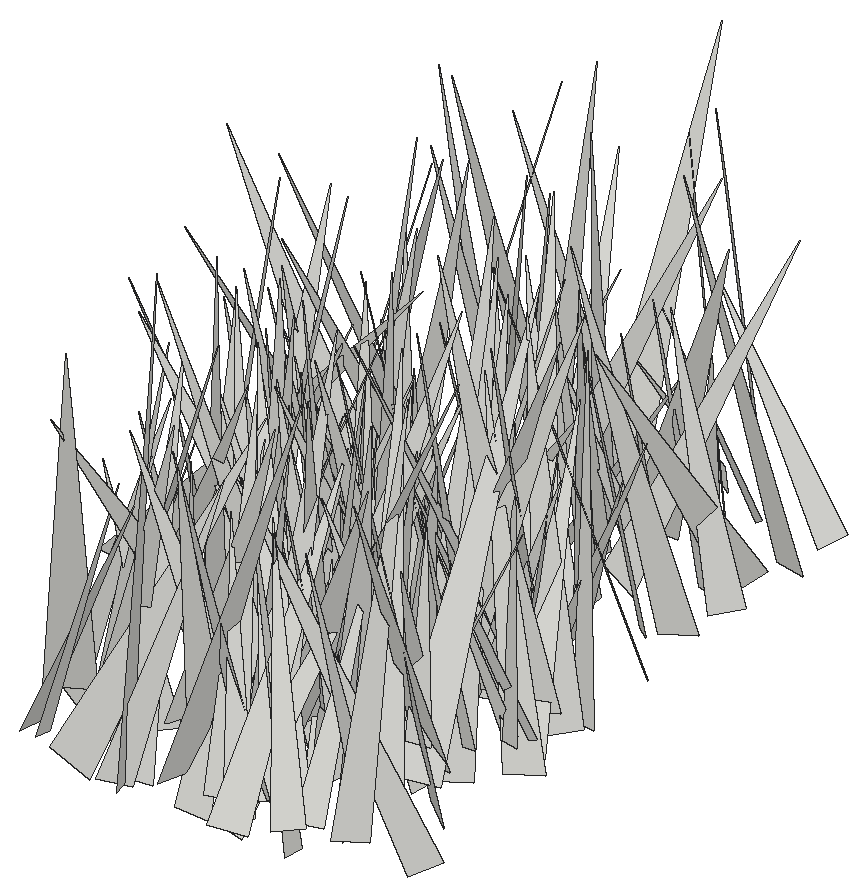
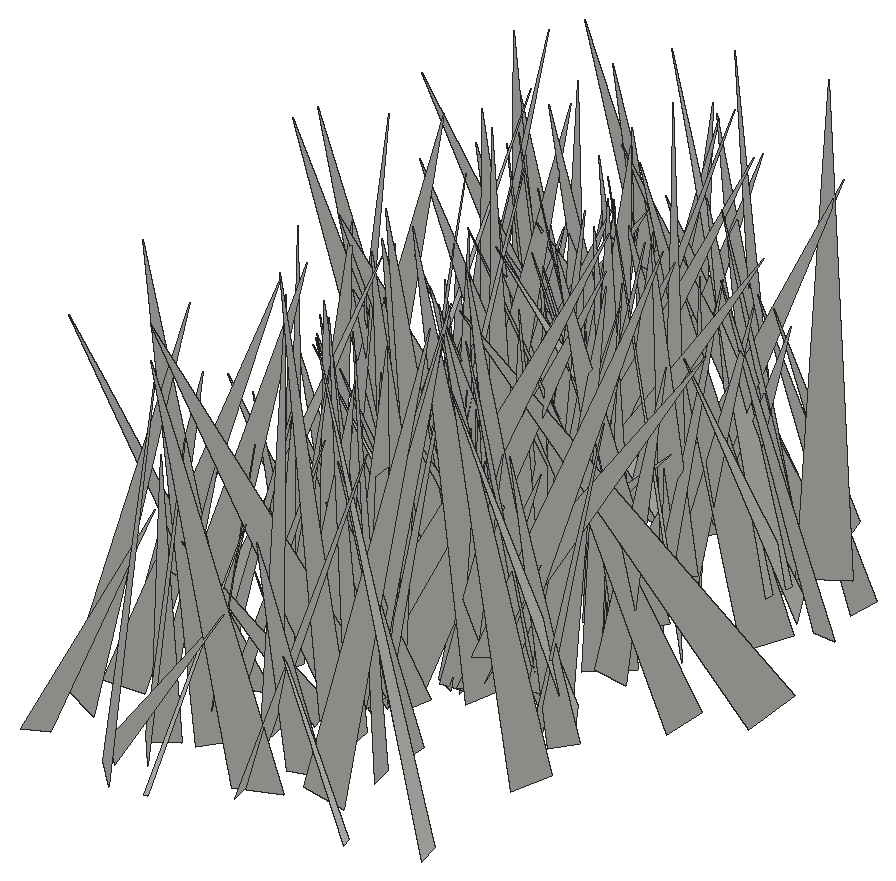
# SketchUp Ruby script. Lengths in inches.
U = 1.inch
M = Sketchup.active_model
def pt(a) = Geom::Point3d.new(a.map { |v| v * U })
def face(e, loops, mat)
  f = e.add_face(loops[0].map { |a| pt(a) })
  loops[1..].each { |l| e.add_face(l.map { |a| pt(a) }).erase! }
  f.material = f.back_material = mat if mat
  f
end
# faces: each face lists its corners as indices into pts; further lists are holes
def faces(e, pts, list, mat = nil) = list.each { |f| face(e, (f[0].is_a?(Array) ? f : [f]).map { |l| l.map { |i| pts[i] } }, mat) }
# xy, xz, yz: faces in a plane at the given z, y or x. An outline is a flat list of corners, or four numbers for a rectangle; further outlines are holes
def ring(l) = l.size == 4 ? [[l[0], l[1]], [l[2], l[1]], [l[2], l[3]], [l[0], l[3]]] : l.each_slice(2).to_a
def flat(e, list, mat, &to3) = list.each { |f| face(e, (f[0].is_a?(Array) ? f : [f]).map { |l| ring(l).map { |u, v| to3.(u, v) } }, mat) }
def xy(e, z, list, mat = nil) = flat(e, list, mat) { |x, y| [x, y, z] }
def xz(e, y, list, mat = nil) = flat(e, list, mat) { |x, z| [x, y, z] }
def yz(e, x, list, mat = nil) = flat(e, list, mat) { |y, z| [x, y, z] }
def lines(e, pts, list) = list.each { |a, b| e.add_line(pt(pts[a]), pt(pts[b])) }
# prism: a flat outline (further loops are holes) pulled along v
def prism(e, loops, v, mat = nil)
  f = face(e, loops, mat); d = Geom::Vector3d.new(v.map { |x| x * U })
  f.pushpull(f.normal.samedirection?(d) ? d.length : -d.length)
end
def box(e, o, s, mat = nil) = prism(e, [[o, [o[0] + s[0], o[1], o[2]], [o[0] + s[0], o[1] + s[1], o[2]], [o[0], o[1] + s[1], o[2]]]], [0, 0, s[2]], mat)
def at(x, y, z, deg = 0) = Geom::Transformation.translation(pt([x, y, z])) * Geom::Transformation.rotation(ORIGIN, Z_AXIS, deg.degrees)
def axes(o, x, y, z) = Geom::Transformation.new([*x, 0, *y, 0, *z, 0, *pt(o).to_a, 1])
def part(name) = M.definitions.add(name)
# library, detail: a bought-in or finely detailed component or shape, given as its bounding box
def library(name, o, s) = part(name).tap { |d| box(d.entities, o, s) }
def detail(e, o, s) = box(e.add_group.entities, o, s)
def put(e, d, t, mat = nil) = e.add_instance(d, t).tap { |i| i.material = mat if mat }
def group(e, t, mat = nil) = e.add_group.tap { |g| g.transformation = t; g.material = mat if mat }.entities
root = M.entities
c1 = part("fur_instance\#9")
p = [[0.8125,0,1.79],[0.67,-0.02,1.48],[0,-0.11,0],[0,0.11,0]]
faces(c1.entities,p,[[0,1,2,3]])
put(root,c1,axes([88.67,204.02,-27.1],[-0.10037,-5.00985,1.67679],[-5.24561,-0.10471,-0.62683],[-0.62754,1.67652,4.9715]))
put(root,c1,axes([86.56,196.72,-28.22],[2.54446,5.11145,1.43196],[5.2695,-2.24073,-1.36501],[0.64019,-1.87187,5.54418]))
put(root,c1,axes([88,208.36,-27.1],[-4.12038,-2.11418,1.50488],[-1.47976,4.23386,1.89649],[2.13184,-1.14743,4.225]))
put(root,c1,axes([83.72,202.71,-27.1],[6.0984,-4.54505,0.22334],[-3.82324,-4.91501,4.37303],[2.46783,3.61705,6.22291]))
put(root,c1,axes([87.83,206.67,-27.1],[5.27233,3.79468,0.9806],[3.62511,-5.34626,1.19781],[-1.48988,0.42019,6.38454]))
put(root,c1,axes([86.71,194.7,-28.22],[4.99939,-0.31235,0.02616],[-0.31267,-4.999,0.06629],[-0.02197,0.06779,5.0087]))
put(root,c1,axes([88.11,195.89,-28.22],[4.4489,2.71988,0.66857],[2.4928,-4.41728,1.38241],[-1.27698,0.85286,5.02786]))
put(root,c1,axes([91.18,206.82,-27.1],[-7.69272,2.37823,1.5322],[2.71051,7.46743,2.01798],[0.8104,-2.40066,7.79498]))
put(root,c1,axes([86.53,203.27,-28.22],[5.89255,-1.31891,0.46121],[-1.38894,-5.74659,1.31223],[-0.15186,1.38261,5.89404]))
put(root,c1,axes([87.44,195.62,-27.1],[4.02071,-6.30995,0.86141],[-6.36147,-4.02715,0.19326],[-0.29869,0.83076,7.47959]))
put(root,c1,axes([87.19,208.02,-27.1],[2.31724,-3.70248,0.25487],[-3.62607,-2.19471,1.08527],[0.79054,0.78602,4.23086]))
put(root,c1,axes([86.52,210.37,-27.1],[7.28234,-1.08518,0.65082],[-1.04869,-7.30325,-0.44316],[-0.70811,-0.34428,7.3494]))
put(root,c1,axes([92.48,206.29,-27.1],[-2.35699,-6.63901,0.53799],[-6.01099,1.87426,-3.2057],[-2.86948,1.52709,6.27339]))
put(root,c1,axes([86.24,215.52,-27.1],[7.20484,3.15988,1.15153],[3.35999,-6.88107,-2.14053],[-0.14588,-2.42624,7.57051]))
put(root,c1,axes([88.13,201.4,-27.1],[5.88152,4.86813,2.28116],[5.13014,-6.09312,-0.22398],[-1.60749,-1.63397,7.63157]))
put(root,c1,axes([88.56,192.9,-27.1],[4.03699,1.00135,1.00845],[0.75439,-4.0837,1.03503],[-1.2044,0.79854,4.02849]))
put(root,c1,axes([89.36,205.97,-27.1],[1.80262,-6.00522,1.15434],[-6.08405,-1.88243,-0.2921],[-0.61598,1.01901,6.26312]))
put(root,c1,axes([90.63,198.56,-28.22],[-1.01611,-5.1437,1.43202],[-5.3112,0.8243,-0.80778],[-0.54728,1.55038,5.1805]))
put(root,c1,axes([89.47,194.375,-27.1],[3.26782,5.25044,1.3347],[5.28581,-3.43164,0.55786],[-1.18691,-0.82697,6.1591]))
put(root,c1,axes([90.27,200.12,-28.22],[-3.05463,-4.97038,1.37571],[-5.09206,3.16016,0.11108],[0.81742,1.11209,5.83293]))
put(root,c1,axes([89.72,201.24,-27.1],[-4.86903,5.31705,1.90275],[5.12727,5.21523,-1.45307],[2.36698,-0.35954,7.06166]))
put(root,c1,axes([91.3,195.46,-27.1],[-1.35537,3.98703,1.26023],[4.07237,0.95801,1.34893],[-0.94888,-1.58348,3.98921]))
put(root,c1,axes([91.07,206.75,-27.1],[-3.67924,-0.76157,0.35539],[-0.68587,3.64327,0.70657],[0.48566,-0.62424,3.6902]))
put(root,c1,axes([90.7,214.8,-27.1],[-1.04582,-7.4675,1.55674],[-7.62212,0.96116,-0.50998],[-0.30029,1.61039,7.52311]))
put(root,c1,axes([90.63,204.97,-28.22],[4.06044,6.49572,1.60929],[6.19974,-4.35997,1.95581],[-2.5194,-0.26008,7.4065]))
put(root,c1,axes([90.6875,198.125,-28.22],[-0.28002,6.79198,1.74012],[7.00527,0.19856,0.35229],[-0.29175,-1.75129,6.78861]))
put(root,c1,axes([91.42,199.84,-28.22],[4.2838,-6.03866,0.74714],[-5.20831,-4.11147,-3.36808],[-3.14598,-1.41597,6.59337]))
put(root,c1,axes([89.03,202.06,-27.1],[-4.56158,-4.36485,4.54967],[-5.17144,5.80258,0.38189],[3.60662,2.79958,6.30192]))
put(root,c1,axes([88.56,216.4375,-27.1],[3.77978,1.93812,0.15141],[1.88384,-3.56988,-1.33157],[0.48001,-1.25124,4.0336]))
put(root,c1,axes([87.59,198.0625,-28.22],[6.5822,-3.48627,0.04021],[-3.46978,-6.5418,0.80411],[0.34104,0.72931,7.40492]))
put(root,c1,axes([90.8,201.92,-27.1],[-3.25997,-4.21096,1.97124],[-4.4396,3.53441,0.20814],[1.38129,1.42168,5.3213]))
put(root,c1,axes([91.86,202.38,-27.1],[-6.39617,-0.72322,1.67284],[-0.5993,6.59982,0.56183],[1.72113,-0.38959,6.41236]))
put(root,c1,axes([90.17,202.17,-28.22],[5.05478,-5.09898,2.04992],[-5.28407,-5.27475,-0.09077],[-1.51011,1.38923,7.17929]))
put(root,c1,axes([91.77,207.32,-27.1],[1.42744,-3.53628,2.17287],[-3.81125,-2.02664,-0.79456],[-1.64348,1.62839,3.72982]))
put(root,c1,axes([91.72,203.55,-28.22],[-4.92159,1.07561,1.43405],[1.22896,5.07505,0.41117],[1.30503,-0.72281,5.02095]))
put(root,c1,axes([91.13,193.9375,-28.22],[-0.62472,6.74476,1.37593],[6.88336,0.62526,0.06028],[0.06565,-1.37569,6.77336]))
put(root,c1,axes([92.85,215.76,-27.1],[-6.22564,-1.43503,0.72375],[-1.44178,6.26598,0.02194],[0.71021,0.14105,6.38885]))
put(root,c1,axes([90.58,198.62,-27.1],[7.19679,1.10507,2.93039],[1.40985,-7.70082,-0.55845],[-2.79655,-1.03845,7.25969]))
put(root,c1,axes([90.63,203.49,-27.1],[4.23333,1.58778,2.03705],[2.11026,-4.38143,-0.97034],[-1.48911,-1.69519,4.41595]))
put(root,c1,axes([92.93,204.93,-28.22],[-6.67208,0.88571,0.68005],[0.61302,6.34873,-2.25421],[0.93335,2.16166,6.3419]))
put(root,c1,axes([87.98,197.04,-27.1],[8.03575,1.73258,0.69022],[1.85682,-7.7181,-2.24381],[-0.17451,-2.34107,7.90825]))
put(root,c1,axes([93.67,209.41,-27.1],[1.68916,7.29229,2.94864],[7.0223,-2.75681,2.79508],[-3.5439,-1.98689,6.94394]))
put(root,c1,axes([90.39,201.42,-27.1],[5.9168,-1.45412,1.7202],[-1.44139,-6.15974,-0.24915],[-1.73089,0.15879,6.08776]))
put(root,c1,axes([89.06,195.42,-28.22],[2.07111,-6.85146,1.31632],[-6.80663,-1.68294,1.94991],[1.53132,1.78604,6.88693]))
put(root,c1,axes([90.87,201.98,-27.1],[-1.22041,-5.00142,1.71972],[-5.19067,1.47111,0.5948],[1.01418,1.51086,5.11369]))
put(root,c1,axes([91.99,214.01,-27.1],[-1.75814,5.2069,0.13379],[5.20853,1.75836,0.01288],[0.0306,-0.13088,5.4957]))
put(root,c1,axes([95.95,198.13,-28.22],[-5.6206,-6.05261,0.8091],[-5.56666,4.62654,-4.06048],[-2.5102,3.29256,7.1929]))
put(root,c1,axes([93.41,207.71,-27.1],[0.03934,-7.1777,0.79174],[-6.87762,-0.27857,-2.18369],[-2.20103,0.74216,6.83757]))
put(root,c1,axes([90.37,205.62,-27.1],[0.14436,6.2225,2.72909],[6.68972,0.34776,-1.14678],[1.18962,-2.71069,6.11762]))
put(root,c1,axes([91.48,196.51,-27.1],[-1.7362,-3.80786,1.79903],[-4.13168,1.91701,0.07019],[0.81577,1.60498,4.18441]))
put(root,c1,axes([91.21,201,-28.22],[2.09335,-3.21544,0.11512],[-3.16402,-2.08217,-0.6229],[-0.58423,-0.24481,3.78592]))
put(root,c1,axes([90.17,212.79,-27.1],[6.17791,2.14602,1.95241],[2.61385,-6.11017,-1.55482],[-1.25898,-2.15507,6.35252]))
put(root,c1,axes([93.86,201.84,-28.22],[-6.45817,-1.9042,0.82118],[-2.02073,6.38203,-1.093],[0.4658,1.28531,6.64374]))
put(root,c1,axes([94.68,200.33,-27.1],[-3.03964,-3.22245,0.08473],[-2.53096,2.3136,-2.80576],[-1.9964,1.97328,3.42802]))
put(root,c1,axes([92.28,203.53,-27.1],[-1.52023,5.3398,1.43684],[5.52962,1.4775,0.35965],[0.03531,-1.48075,5.54032]))
put(root,c1,axes([90.29,211.18,-27.1],[4.64255,0.07182,0.51653],[0.0806,-4.67045,-0.07504],[-0.51523,-0.08349,4.6425]))
put(root,c1,axes([95,206.625,-27.1],[-3.02685,-7.70536,1.30124],[-7.48247,2.45538,-2.86554],[-2.25353,2.19686,7.76679]))
put(root,c1,axes([92.36,192.05,-27.1],[-7.10447,-2.39928,3.44832],[-3.25719,7.42464,-1.54476],[2.65295,2.69055,7.33783]))
put(root,c1,axes([92.16,207.35,-27.1],[-1.43466,-3.23484,0.82707],[-3.31328,1.49057,0.08262],[0.41278,0.72144,3.53774]))
put(root,c1,axes([90.76,207.02,-27.1],[7.15421,-1.9799,2.12173],[-2.22149,-7.36827,0.61487],[-1.86728,1.18029,7.39761]))
put(root,c1,axes([89.07,193.55,-28.22],[0.42432,7.03314,2.02201],[6.63788,0.48281,-3.07232],[3.08094,-2.00885,6.34082]))
put(root,c1,axes([93.4,210.47,-27.1],[-1.73003,-6.76572,2.01517],[-7.01807,1.42401,-1.24409],[-0.76325,2.2419,6.8717]))
put(root,c1,axes([94.2,195.89,-27.1],[-0.66678,7.09806,0.59701],[6.83624,0.46921,2.05647],[-2.00116,-0.76214,6.82627]))
put(root,c1,axes([94.1,203.72,-28.22],[-3.14834,2.92622,0.07201],[2.87738,3.07451,0.86494],[-0.53726,-0.68166,4.21031]))
put(root,c1,axes([95.25,199.83,-28.22],[-7.87957,1.88276,1.17896],[2.17634,7.41366,2.70618],[0.44527,-2.91806,7.63603]))
put(root,c1,axes([94.67,198.18,-27.1],[-7.8071,-1.03462,1.04066],[-0.93299,7.84786,0.80297],[1.13267,-0.66693,7.83431]))
put(root,c1,axes([92.92,209.3,-27.1],[-2.78076,-3.999,1.01738],[-3.97731,2.92434,0.62365],[1.09912,0.46468,4.83071]))
put(root,c1,axes([91.3125,198.9,-28.22],[5.1332,2.66859,0.80867],[2.72409,-5.16107,-0.26035],[-0.59552,-0.60587,5.77956]))
put(root,c1,axes([91.71,195.98,-28.22],[6.02604,4.35688,0.13616],[4.14402,-5.7981,2.12678],[-1.35204,1.64734,7.12547]))
put(root,c1,axes([92.08,211.55,-27.1],[6.17707,1.48648,1.9777],[1.80034,-6.34915,-0.85095],[-1.69697,-1.32504,6.29616]))
put(root,c1,axes([92.28,205.46,-27.1],[3.64013,-0.49009,0.65042],[-0.33955,-3.62113,-0.82821],[-0.74023,-0.74902,3.57838]))
put(root,c1,axes([92.1,191.9,-27.1],[4.14579,-2.60609,2.17076],[-3.31381,-3.84297,1.71517],[-0.72292,2.67047,4.58667]))
put(root,c1,axes([92.86,211.54,-27.1],[2.51079,7.35519,2.45383],[7.71335,-2.63218,-0.00261],[-0.79014,-2.32314,7.77193]))
put(root,c1,axes([92.45,215.7,-27.1],[-1.03239,7.59334,1.92082],[7.72051,1.31303,-1.04105],[1.31985,-1.74108,7.59215]))
put(root,c1,axes([94.75,195.29,-27.1],[-5.48359,2.23586,1.70204],[2.68404,5.27249,1.72124],[0.83185,-2.27324,5.66623]))
put(root,c1,axes([93.9,199.51,-27.1],[3.52477,-3.78027,2.43443],[-3.94318,-4.08529,-0.63451],[-2.1606,1.28874,5.1295]))
put(root,c1,axes([96.17,197.18,-27.1],[-1.67581,5.69721,1.32161],[5.39716,0.9769,2.63242],[-2.25291,-1.89755,5.32325]))
put(root,c1,axes([94.71,199.63,-27.1],[-3.5063,-5.04513,2.56803],[-5.65565,3.25438,-1.32851],[0.24851,2.88062,5.99854]))
put(root,c1,axes([92.49,209.21,-27.1],[3.64505,-0.39812,0.27738],[-0.20845,-3.18305,-1.82936],[-0.43816,-1.79764,3.17779]))
put(root,c1,axes([93.27,201.86,-28.22],[4.67368,1.9817,0.84614],[1.46066,-4.3994,2.23565],[-1.58416,1.79011,4.55767]))
put(root,c1,axes([95.12,198.55,-27.1],[-3.33504,1.53851,0.16438],[1.54705,3.32218,0.29368],[0.02564,-0.33558,3.66104]))
put(root,c1,axes([95.26,201.24,-28.22],[0.65103,4.23875,0.31259],[3.78552,-0.72206,1.9071],[-1.9325,0.01355,3.84107]))
put(root,c1,axes([93.59,205.57,-27.1],[-2.68709,-2.60275,1.28992],[-2.48203,2.97011,0.82256],[1.50922,0.25052,3.6494]))
put(root,c1,axes([93.89,193.41,-28.22],[0.04484,6.03011,0.93276],[6.10111,-0.02998,-0.09948],[0.09373,-0.93336,6.02946]))
put(root,c1,axes([93.67,194.61,-27.1],[3.36896,-5.0045,1.18358],[-5.04079,-3.49374,-0.42432],[-1.01802,0.73793,6.01788]))
put(root,c1,axes([94.76,199.71,-28.22],[-5.05417,-1.27819,2.14403],[-1.86511,5.15169,-1.32541],[1.65892,1.89778,5.04199]))
put(root,c1,axes([94.18,212.875,-27.1],[-6.46976,-1.55499,2.98827],[-1.52534,7.12153,0.40334],[3.00351,0.26714,6.64177]))
put(root,c1,axes([92.61,198.42,-27.1],[3.5807,5.01538,0.32607],[5.01642,-3.54168,-0.61141],[0.30977,-0.61982,6.13202]))
put(root,c1,axes([91.86,195.84,-27.1],[3.71453,-6.09838,0.78607],[-6.05056,-3.46164,1.73599],[1.09493,1.55972,6.92635]))
put(root,c1,axes([93.44,201.57,-27.1],[4.01305,-1.4697,0.35123],[-1.33059,-3.90931,-1.15533],[-0.71618,-0.97223,4.11458]))
put(root,c1,axes([93.33,208.65,-27.1],[3.21105,-3.45107,0.18225],[-3.45172,-3.21492,-0.06213],[-0.16965,0.09106,4.71348]))
put(root,c1,axes([92.04,208.89,-27.1],[2.63596,-3.80697,0.02165],[-3.40971,-2.34911,2.07299],[1.69332,1.196,4.14053]))
put(root,c1,axes([93.87,196.59,-28.22],[3.27247,4.57721,0.86039],[4.6176,-3.3258,0.13012],[-0.60735,-0.62316,5.62521]))
put(root,c1,axes([94.32,201.8,-28.22],[7.55648,0.00384,2.83421],[0.13477,-8.06186,-0.34839],[-2.831,-0.37353,7.54844]))
put(root,c1,axes([96.33,208.05,-27.1],[-2.8304,4.89567,0.80261],[4.94903,2.72215,0.8485],[-0.34477,-1.11592,5.59096]))
put(root,c1,axes([95.92,194.07,-27.1],[-2.42816,-5.42807,1.43938],[-5.61543,2.33238,-0.67728],[-0.05217,1.5899,5.90772]))
put(root,c1,axes([95.34,193.2,-27.1],[-1.64071,6.20292,1.41522],[6.35653,1.66047,0.09149],[0.27128,-1.39198,6.41559]))
put(root,c1,axes([97.22,216.5,-27.1],[-2.6027,-3.00196,0.39616],[-2.70686,2.07255,-2.07851],[-1.35707,1.62343,3.38609]))
put(root,c1,axes([94.85,217.9,-27.1],[-2.93741,-3.09466,0.01129],[-2.71699,2.58635,2.03327],[1.48156,-1.39259,3.75115]))
put(root,c1,axes([96.63,201.31,-27.1],[1.14957,-5.99203,1.40359],[-5.68779,-1.57972,-2.08556],[-2.35023,0.89221,5.73379]))
put(root,c1,axes([96.74,194.3,-27.1],[-5.17368,4.83178,0.63052],[4.85594,5.1888,0.08232],[0.40437,-0.49072,7.07858]))
put(root,c1,axes([95.13,200.06,-28.22],[-5.22484,3.83291,1.4033],[3.4058,5.3502,-1.93269],[2.24967,0.80218,6.18505]))
put(root,c1,axes([96.63,202.24,-28.22],[-1.35927,-4.19334,1.10265],[-4.18909,0.97193,-1.4678],[-1.11869,1.45561,4.1566]))
put(root,c1,axes([93.76,211.02,-27.1],[3.8069,0.05751,0.20355],[-0.0416,-3.39391,1.73693],[-0.20739,1.73647,3.38805]))
put(root,c1,axes([96.42,203.39,-28.22],[-5.73221,-5.07274,1.73381],[-5.23258,5.8463,-0.19467],[1.1657,1.29813,7.652]))
put(root,c1,axes([96.74,205.14,-28.22],[-6.05277,2.56522,0.71834],[2.46544,6.06973,-0.90131],[1.00895,0.55714,6.51184]))
put(root,c1,axes([96.5,215.78,-27.1],[3.70498,4.05955,2.96614],[3.93602,-4.63444,1.42637],[-3.1282,-1.02317,5.30776]))
put(root,c1,axes([93.35,200.82,-27.1],[2.79379,4.96818,0.70977],[4.95175,-2.59669,-1.31495],[0.8165,-1.25148,5.54607]))
put(root,c1,axes([94.49,195.61,-27.1],[5.43956,-0.0104,1.6458],[0.01524,-5.68242,-0.08629],[-1.64576,-0.087,5.43889]))
put(root,c1,axes([93.84,199.47,-28.22],[7.49694,-1.26912,1.50095],[-0.87324,-7.45265,-1.93987],[-1.76095,-1.70734,7.35199]))
put(root,c1,axes([95.42,203.66,-27.1],[-1.01475,7.09695,1.79918],[7.31311,1.06925,-0.09303],[0.3496,-1.76734,7.16853]))
put(root,c1,axes([94.83,203.32,-27.1],[-1.17903,-5.46423,1.73554],[-5.62366,1.44698,0.7353],[1.11548,1.51937,5.54141]))
put(root,c1,axes([96.32,206.78,-27.1],[-3.98192,5.65644,1.02142],[5.69703,4.04883,-0.21229],[0.76316,-0.7113,6.91418]))
put(root,c1,axes([93.08,210.08,-27.1],[6.18283,-3.26103,2.17206],[-3.91127,-5.37775,3.05962],[-0.2327,3.74499,6.28493]))
put(root,c1,axes([95.24,202.79,-28.22],[4.16098,5.56887,0.17793],[5.30628,-4.02846,1.99315],[-1.69922,1.05685,6.65984]))
put(root,c1,axes([96.46,192.43,-27.1],[-4.11869,2.39634,0.55767],[2.352,4.15398,-0.47915],[0.72219,0.13795,4.74094]))
put(root,c1,axes([96.5,209.36,-27.1],[-5.34365,-1.01248,1.41227],[-1.15776,5.47992,-0.452],[1.29585,0.72082,5.4199]))
put(root,c1,axes([96.1875,212.26,-27.1],[-4.24869,-0.73201,1.00331],[-0.4187,4.21079,1.29914],[1.16925,-1.15205,4.11089]))
put(root,c1,axes([96.05,196.61,-28.22],[-1.12302,3.48075,0.37457],[3.50037,1.10997,0.18007],[-0.0574,-0.41163,3.65299]))
put(root,c1,axes([93.34,193.41,-27.1],[7.44021,-1.05618,0.97458],[-1.13327,-7.472,0.55406],[-0.88376,0.68976,7.49435]))
put(root,c1,axes([93.96,199.375,-27.1],[-0.17372,7.00266,1.70424],[6.95108,0.61311,-1.81067],[1.90374,-1.5996,6.76675]))
put(root,c1,axes([94.92,196.51,-27.1],[4.55576,-0.64185,1.19418],[-0.37344,-4.61891,-1.05794],[-1.3033,-0.92017,4.47746]))
put(root,c1,axes([94.17,203.84,-28.22],[1.86244,4.7215,0.55373],[4.68693,-1.72429,-1.06173],[0.79484,-0.89561,4.96326]))
put(root,c1,axes([94.89,211.63,-27.1],[4.79188,-1.27621,1.00499],[-1.01396,-4.79557,-1.25507],[-1.26909,-0.98723,4.79746]))
put(root,c1,axes([95.79,194.46,-27.1],[0.08321,7.29137,1.2347],[7.39423,-0.10178,0.10277],[-0.11831,-1.23331,7.29112]))
put(root,c1,axes([94.91,201.54,-27.1],[4.77554,-0.30271,1.03368],[-0.19329,-4.86277,-0.53104],[-1.0596,-0.47722,4.75556]))
put(root,c1,axes([97.125,198.25,-27.1],[-5.33411,1.7362,0.45715],[1.45522,5.02033,-2.08679],[1.05153,1.85957,5.20696]))
put(root,c1,axes([96.54,217.64,-27.1],[-4.69837,-4.55111,2.1601],[-4.81656,4.92378,-0.10244],[1.47629,1.58022,6.5404]))
put(root,c1,axes([95.88,204.31,-28.22],[-2.76968,5.79414,2.34049],[6.07448,3.09716,-0.47899],[1.46654,-1.88589,6.4042]))
put(root,c1,axes([94.44,203.12,-28.22],[4.81991,2.46867,0.79438],[2.57067,-4.76928,-0.77622],[-0.3421,-1.05666,5.35942]))
put(root,c1,axes([96.51,197,-27.1],[-2.7828,-3.97435,1.2381],[-4.07565,2.90431,0.16237],[0.84701,0.91751,4.84903]))
put(root,c1,axes([97.74,193.46,-28.22],[-5.27526,-0.92635,0.94955],[-1.13263,5.17215,-1.24665],[0.69057,1.40673,5.20887]))
put(root,c1,axes([96.72,200.49,-27.1],[1.44091,-6.85532,1.40735],[-6.89305,-1.6385,-0.92385],[-1.20912,1.1714,6.94393]))
put(root,c1,axes([95.08,202.77,-27.1],[3.8804,-2.67072,0.47699],[-2.66948,-3.90717,-0.15997],[-0.48385,0.13783,4.70793]))
put(root,c1,axes([96.59,191.73,-27.1],[-4.56686,4.07542,0.09193],[3.68922,4.19072,-2.51023],[1.73411,1.8173,5.58247]))
put(root,c1,axes([96.7,212.46,-27.1],[-3.36264,-2.39418,1.21792],[-2.41208,3.55006,0.31902],[1.18208,0.43333,4.11555]))
put(root,c1,axes([96.21,196.32,-28.22],[4.33311,5.30156,2.10924],[5.44411,-4.63436,0.46433],[-1.70794,-1.32191,6.83131]))
put(root,c1,axes([95.23,193.35,-28.22],[-0.37436,5.47936,0.25355],[5.20879,0.43477,-1.70506],[1.71934,-0.12411,5.22075]))
put(root,c1,axes([97.23,196.5625,-27.1],[-3.6032,0.74818,1.09352],[0.87855,3.72087,0.34907],[0.99182,-0.57787,3.66346]))
put(root,c1,axes([98,192.89,-27.1],[-3.61656,3.24074,0.55892],[3.26072,3.64166,-0.01623],[0.42715,-0.36083,4.85609]))
put(root,c1,axes([97.56,202.47,-27.1],[-5.57513,-2.9786,1.92177],[-3.03694,5.86084,0.2736],[1.82819,0.65252,6.315]))
put(root,c1,axes([98.7,199.79,-28.22],[-7.37463,3.18086,0.67882],[2.84062,7.11825,-2.49505],[1.58417,2.04365,7.63399]))
put(root,c1,axes([97.67,204.62,-27.1],[-5.6893,-5.57398,0.54513],[-5.22917,5.56506,2.3282],[2.00554,-1.30211,7.61688]))
put(root,c1,axes([94.6,197.36,-27.1],[3.61715,-5.66391,0.01487],[-5.50634,-3.51236,1.58351],[1.3268,0.86448,6.53117]))
put(root,c1,axes([96.21,209.375,-27.1],[6.38697,0.74513,2.00431],[1.2691,-6.40204,-1.66407],[-1.72101,-1.95564,6.21124]))
put(root,c1,axes([98.3,199.27,-28.22],[-4.94323,1.53486,1.76986],[2.06825,4.80019,1.61379],[1.10026,-2.12747,4.91803]))
put(root,c1,axes([96.35,215.05,-27.1],[1.68114,-3.92704,0.2758],[-3.91607,-1.63754,0.5539],[0.40264,0.46985,4.23569]))
put(root,c1,axes([98.6,212.18,-27.1],[-2.6227,-3.62693,1.52989],[-3.9333,2.34177,-1.19122],[-0.15598,1.93268,4.31442]))
put(root,c1,axes([98.75,209.01,-27.1],[-3.38469,-3.26483,1.22467],[-3.48648,3.19729,-1.11215],[0.05857,1.65326,4.56929]))
put(root,c1,axes([94.81,195.37,-28.22],[8.11647,0.24258,0.67526],[0.10402,-7.98511,1.61836],[-0.70993,1.60345,7.95719]))
put(root,c1,axes([99.28,203.17,-27.1],[1.07794,-7.21694,3.00432],[-7.53412,-1.768,-1.54384],[-2.08502,2.65746,7.13181]))
put(root,c1,axes([101.48,195.15,-28.22],[-2.20634,6.02099,1.75888],[5.48729,0.94934,3.63349],[-3.03901,-2.65713,5.28374]))
put(root,c1,axes([99.75,216.89,-27.1],[-4.14397,2.00475,0.46664],[2.04964,3.92263,1.34951],[-0.1891,-1.41534,4.40117]))
put(root,c1,axes([100.23,201.72,-27.1],[-2.15609,-3.98258,0.83043],[-3.73233,1.56246,-2.1972],[-1.61872,1.70208,3.96005]))
put(root,c1,axes([95.04,214.08,-27.1],[3.43044,-6.71204,0.2285],[-6.5076,-3.25868,1.97581],[1.6598,1.09595,7.27431]))
put(root,c1,axes([99.125,200.17,-27.1],[0.98464,3.25356,1.70885],[3.23357,-1.6077,1.19779],[-1.74639,-1.14237,3.18127]))
put(root,c1,axes([98.1,195.21,-28.22],[4.10758,4.73433,2.04961],[4.7509,-4.49256,0.85604],[-2.01089,-0.9434,6.20913]))
put(root,c1,axes([100.34,207.11,-27.1],[-4.77204,-4.71706,0.72174],[-4.75307,4.60775,-1.31181],[-0.42413,1.43592,6.58044]))
put(root,c1,axes([99.67,209.57,-27.1],[0.21483,-6.37799,2.26736],[-6.52313,-0.80094,-1.63496],[-1.80789,2.13204,6.16862]))
put(root,c1,axes([98.875,196.09,-27.1],[-4.66477,5.25581,1.41142],[5.28211,4.8201,-0.49149],[1.30953,-0.72026,7.01013]))
put(root,c1,axes([95.3,203.61,-27.1],[6.73019,-3.63445,0.24466],[-3.63894,-6.68481,0.79754],[0.16506,0.81773,7.60715]))
put(root,c1,axes([98.3,193.48,-27.1],[-2.89622,3.26829,0.45856],[3.08153,2.89643,-1.18106],[1.18158,0.4572,4.20415]))
put(root,c1,axes([96.75,197.42,-27.1],[1.17018,-6.95871,1.51726],[-7.0392,-0.89595,1.31981],[1.08411,1.69372,6.93189]))
put(root,c1,axes([99.1,197.6,-27.1],[-6.13074,4.86156,0.06985],[4.48302,5.69573,-2.94734],[1.88206,2.26926,7.24803]))
put(root,c1,axes([97.26,203.4,-27.1],[3.48145,-1.92251,0.90917],[-2.10367,-3.36896,0.93158],[-0.31179,1.26381,3.86636]))
put(root,c1,axes([99.78,214.79,-27.1],[-2.51805,-6.35566,1.6356],[-6.55451,2.34778,-0.96776],[-0.32873,1.87181,6.76746]))
put(root,c1,axes([99.41,204.16,-28.22],[-5.4066,3.91291,1.98693],[4.14231,5.59139,0.26032],[1.44915,-1.38406,6.66892]))
put(root,c1,axes([96.64,200.2,-28.22],[4.2362,2.18763,0.04516],[2.18011,-4.21144,-0.49393],[0.18673,-0.4595,4.74206]))
put(root,c1,axes([96.17,211.04,-27.1],[1.82211,6.46965,0.85286],[6.26515,-1.48669,-2.10749],[1.8253,-1.35544,6.38239]))
put(root,c1,axes([97.7,205.43,-27.1],[-3.32814,-6.39102,1.50803],[-6.07577,3.63841,2.01068],[2.49085,0.3356,6.91945]))
put(root,c1,axes([98.94,195.37,-27.1],[-4.40075,-1.21691,1.44212],[-0.98766,4.60363,0.87078],[1.60783,-0.50284,4.4821]))
put(root,c1,axes([97.55,200.34,-28.22],[4.75134,-2.11282,0.36953],[-1.90852,-4.57438,-1.61505],[-0.97883,-1.33672,4.94275]))
put(root,c1,axes([99.64,198.01,-28.22],[4.25123,5.18566,4.75994],[6.35301,-5.22113,0.01405],[-3.03108,-3.67013,6.70551]))
put(root,c1,axes([96.38,202.22,-27.1],[3.6811,-6.05089,2.6185],[-6.53456,-2.94932,2.37094],[0.87715,3.42178,6.67401]))
put(root,c1,axes([97.42,207.51,-27.1],[3.61055,-0.61097,0.20103],[-0.59508,-3.6081,-0.27795],[-0.24409,-0.24103,3.65131]))
put(root,c1,axes([99.8,201.875,-28.22],[-0.66847,-3.61729,0.84651],[-3.58891,0.40659,-1.09666],[-0.95975,0.99906,3.51127]))
put(root,c1,axes([100.16,201.53,-28.22],[-2.02202,5.92033,1.45384],[6.05855,1.78151,1.17164],[-0.67672,-1.74024,6.14542]))
put(root,c1,axes([98.2,203.8,-27.1],[3.88099,1.49769,1.22771],[1.56049,-4.04689,0.00388],[-1.14683,-0.43823,4.15995]))
put(root,c1,axes([98.91,197.94,-27.1],[-3.06481,2.41196,1.362],[2.48233,3.29293,-0.24563],[1.22908,-0.63618,3.89234]))
put(root,c1,axes([99.69,204.97,-28.22],[1.64216,5.46326,1.64146],[5.44457,-2.0108,1.24565],[-1.70244,-1.16093,5.56707]))
put(root,c1,axes([99.48,202.49,-28.22],[-1.13883,5.42731,0.08742],[5.42427,1.13458,0.2244],[-0.2017,-0.13157,5.54096]))
put(root,c1,axes([99.89,193.51,-27.1],[-6.30964,2.41528,1.06239],[1.96226,6.1361,-2.29599],[1.76402,1.81341,6.35402]))
put(root,c1,axes([97.88,205.47,-27.1],[4.13014,0.16234,0.60229],[0.00137,-4.03539,1.07832],[-0.62379,1.06603,3.99019]))
put(root,c1,axes([99.95,211.54,-27.1],[-3.61147,3.35043,1.62323],[3.67501,3.56996,0.80783],[0.59541,-1.71259,4.85958]))
put(root,c1,axes([98.87,198.81,-27.1],[-0.42981,-6.03201,0.26249],[-6.01913,0.44871,0.45551],[0.47339,0.22867,6.03012]))
put(root,c1,axes([99.93,201.14,-27.1],[1.9045,4.44389,1.45881],[4.34306,-2.26488,1.22946],[-1.73613,-0.79091,4.67587]))
put(root,c1,axes([99.37,213.28,-27.1],[4.98513,-4.06782,0.78587],[-3.3159,-4.65458,-3.05875],[-2.48386,-1.95039,5.66063]))
